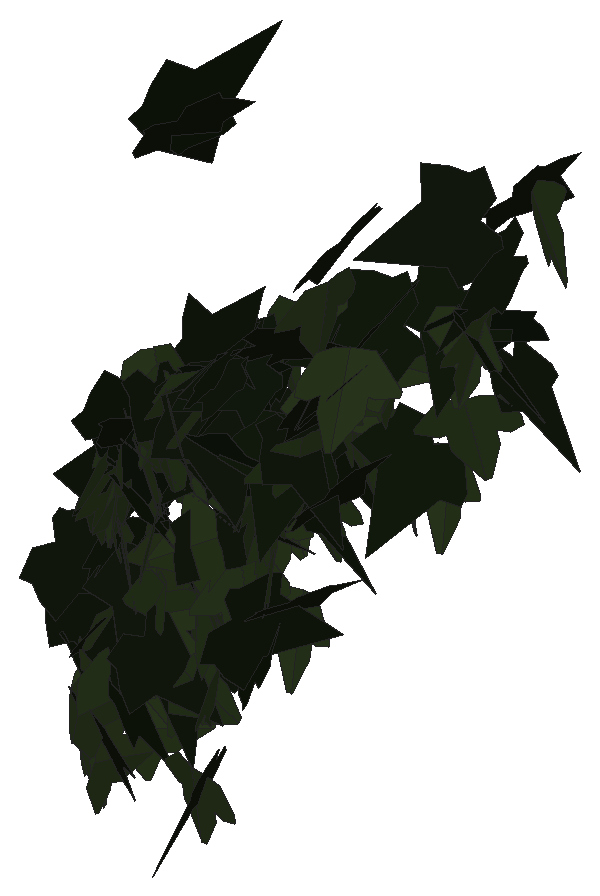
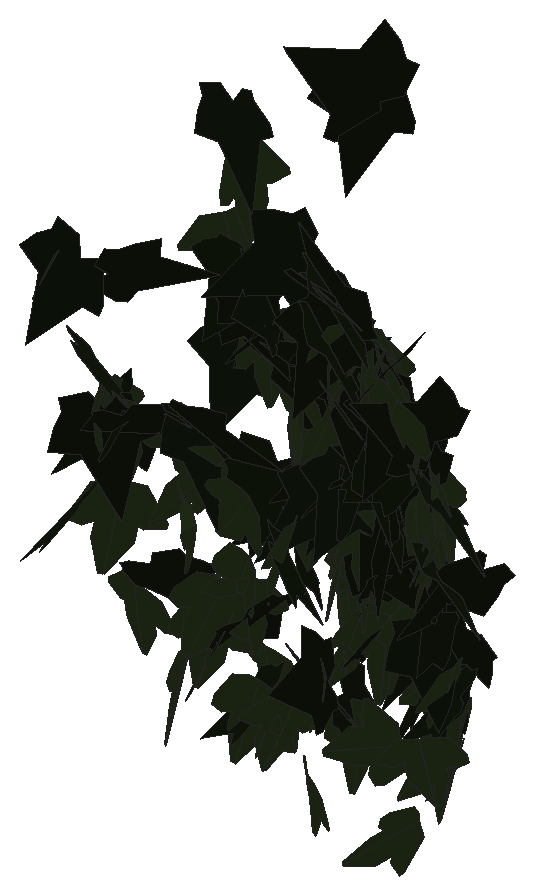
# SketchUp Ruby script. Lengths in inches.
U = 1.inch
M = Sketchup.active_model
def pt(a) = Geom::Point3d.new(a.map { |v| v * U })
def face(e, loops, mat)
  f = e.add_face(loops[0].map { |a| pt(a) })
  loops[1..].each { |l| e.add_face(l.map { |a| pt(a) }).erase! }
  f.material = f.back_material = mat if mat
  f
end
# faces: each face lists its corners as indices into pts; further lists are holes
def faces(e, pts, list, mat = nil) = list.each { |f| face(e, (f[0].is_a?(Array) ? f : [f]).map { |l| l.map { |i| pts[i] } }, mat) }
# xy, xz, yz: faces in a plane at the given z, y or x. An outline is a flat list of corners, or four numbers for a rectangle; further outlines are holes
def ring(l) = l.size == 4 ? [[l[0], l[1]], [l[2], l[1]], [l[2], l[3]], [l[0], l[3]]] : l.each_slice(2).to_a
def flat(e, list, mat, &to3) = list.each { |f| face(e, (f[0].is_a?(Array) ? f : [f]).map { |l| ring(l).map { |u, v| to3.(u, v) } }, mat) }
def xy(e, z, list, mat = nil) = flat(e, list, mat) { |x, y| [x, y, z] }
def xz(e, y, list, mat = nil) = flat(e, list, mat) { |x, z| [x, y, z] }
def yz(e, x, list, mat = nil) = flat(e, list, mat) { |y, z| [x, y, z] }
def lines(e, pts, list) = list.each { |a, b| e.add_line(pt(pts[a]), pt(pts[b])) }
# prism: a flat outline (further loops are holes) pulled along v
def prism(e, loops, v, mat = nil)
  f = face(e, loops, mat); d = Geom::Vector3d.new(v.map { |x| x * U })
  f.pushpull(f.normal.samedirection?(d) ? d.length : -d.length)
end
def box(e, o, s, mat = nil) = prism(e, [[o, [o[0] + s[0], o[1], o[2]], [o[0] + s[0], o[1] + s[1], o[2]], [o[0], o[1] + s[1], o[2]]]], [0, 0, s[2]], mat)
def at(x, y, z, deg = 0) = Geom::Transformation.translation(pt([x, y, z])) * Geom::Transformation.rotation(ORIGIN, Z_AXIS, deg.degrees)
def axes(o, x, y, z) = Geom::Transformation.new([*x, 0, *y, 0, *z, 0, *pt(o).to_a, 1])
def part(name) = M.definitions.add(name)
# library, detail: a bought-in or finely detailed component or shape, given as its bounding box
def library(name, o, s) = part(name).tap { |d| box(d.entities, o, s) }
def detail(e, o, s) = box(e.add_group.entities, o, s)
def put(e, d, t, mat = nil) = e.add_instance(d, t).tap { |i| i.material = mat if mat }
def group(e, t, mat = nil) = e.add_group.tap { |g| g.transformation = t; g.material = mat if mat }.entities
root = M.entities
M.materials.add("efeu1").color = [18, 25, 13]
M.materials.add("efeu2").color = [43, 57, 29]
c1 = part("ivyleaf_10")
p = [[0,0.5,-0.03],[-0.0625,2.02,-0.43],[-0.19,2.01,-0.46],[-0.54,1.05,-0.29],[-0.52,0.625,-0.18],[-0.83,0.76,-0.28],
  [-1.16,0.64,-0.33],[-1.15,0.33,-0.24],[-0.77,-0.39,0.02],[-0.3,-0.51,0.16],[0.04,-0.48,0.23],[-0.02,2.01,-0.4375],
  [-0.06,2.01,-0.43],[0.04,-0.49,0.23],[0.67,-0.49,0.14],[1.38,0.36,-0.2],[1.375,0.51,-0.24],[0.81,0.65,-0.19],
  [0.62,0.59,-0.15],[0.6,1.09,-0.28],[0.5,1.23,-0.31]]
faces(c1.entities,p,[[0,1,2,3,4,5,6,7,8,9,10],[11,12,0,13,14,15,16,17,18,19,20]],"efeu2")
c2 = part("ivyleaf_9")
p = [[1.54,2.16,1.25],[1.36,2.04,1.19],[-0.21,0.99,0.68],[-0.71,1.11,0.82],[-0.85,0.86,0.67],[-0.8,0.17,0.21],
  [-0.9,-0.01,0.1],[-0.67,-0.16,-0.02],[-0.08,-0.08,-0.05],[-0.03,-0.6,-0.4],[0.65,-0.88,-0.66],[0.83,-0.6,-0.49],
  [1.29,-0.42,-0.43],[1.8125,-0.07,-0.26],[1.21,0.44,0.15]]
faces(c2.entities,p,[[0,1,2,3,4,5,6,7,8,9,10,11,12,13,14]],"efeu1")
put(root,c1,axes([559.02,133.74,220.0625],[-0.14078,-0.88216,-0.06887],[0.00264,0.06931,-0.89328],[0.88484,-0.14056,-0.00829]))
put(root,c2,axes([556.01,133.8125,216.23],[-0.26742,-0.68197,-0.50877],[0.17433,0.47808,-0.73246],[0.83279,-0.31907,-0.01004]))
put(root,c1,axes([555.16,133.6,216.0625],[-0.46039,0.75729,-0.00295],[-0.00102,-0.00407,-0.88625],[-0.7573,-0.46038,0.00299]))
put(root,c2,axes([554.58,133.77,216.25],[0.44166,-0.72964,-0.25832],[-0.05083,0.26943,-0.84793],[0.77235,0.43497,0.09191]))
put(root,c2,axes([553.01,133.48,207.98],[0.77653,-0.04593,-0.47015],[-0.46839,0.04255,-0.77778],[0.06131,0.90677,0.01268]))
put(root,c2,axes([556.24,133.74,215.02],[0.44606,-0.24546,0.70342],[0.69118,-0.16966,-0.4975],[0.27807,0.81547,0.10823]))
put(root,c2,axes([556.68,133.75,217.57],[-0.7001,0.49631,0.19101],[-0.23436,-0.00448,-0.84735],[-0.47737,-0.72567,0.13587]))
put(root,c2,axes([555.56,133.26,223.17],[0.31745,0.86349,0.0264],[0.0086,0.02496,-0.92],[-0.86385,0.31757,0.00054]))
put(root,c1,axes([555.84,133.78,213.01],[-0.41657,0.26358,0.71128],[-0.7577,-0.18299,-0.37595],[0.03589,-0.80372,0.31886]))
put(root,c1,axes([554.58,133.89,216],[0.68612,-0.55,-0.06522],[-0.05978,0.02969,-0.87924],[0.55061,0.68858,-0.01419]))
put(root,c2,axes([554.49,133.53,210.3],[0.30628,-0.50665,-0.6268],[-0.10287,0.64048,-0.56797],[0.79937,0.27654,0.16706]))
put(root,c1,axes([559.5,133.85,218.39],[0.57533,0.6599,-0.15884],[-0.14364,-0.08513,-0.87397],[-0.66337,0.59075,0.05149]))
put(root,c2,axes([557.15,134,217.61],[-0.83228,0.17303,0.21694],[-0.22414,-0.01484,-0.84808],[-0.16359,-0.85996,0.05829]))
put(root,c1,axes([554.92,133.88,216.13],[0.05452,-0.88445,-0.07136],[-0.01495,0.07057,-0.88607],[0.8872,0.05554,-0.01054]))
put(root,c1,axes([554.7,133.78,215.36],[-0.86039,0.19813,-0.04154],[0.02888,-0.0594,-0.88141],[-0.20037,-0.85934,0.05135]))
put(root,c2,axes([556.59,133.5,217.71],[-0.36519,0.75552,0.27273],[-0.19522,0.20713,-0.83519],[-0.77916,-0.40601,0.08143]))
put(root,c1,axes([555.77,134.02,215.96],[0.01771,-0.87373,0.07357],[0.04283,-0.07263,-0.87294],[0.87578,0.02123,0.04121]))
put(root,c1,axes([553.21,133.18,208.43],[-0.01588,-0.12607,-0.94432],[0.22937,0.91617,-0.12617],[0.92468,-0.22942,0.01508]))
put(root,c1,axes([558.2,133.92,215.96],[-0.29422,-0.83577,-0.04837],[0.01575,0.04574,-0.88605],[0.83702,-0.29465,-0.00033]))
put(root,c2,axes([557.0625,133.25,211.8],[0.18463,0.11111,-0.87116],[-0.14229,0.88223,0.08236],[0.86662,0.12118,0.19912]))
put(root,c2,axes([555.51,134.36,207.25],[-0.4534,0.18215,-0.71547],[0.52437,-0.5116,-0.46255],[-0.51972,-0.67509,0.15749]))
put(root,c2,axes([557.71,134.3,215.82],[-0.62927,-0.54802,-0.2724],[0.25922,0.11524,-0.83067],[0.55437,-0.67594,0.07922]))
put(root,c1,axes([553.04,134.125,213.8],[0.68555,-0.47728,0.27133],[0.27945,-0.07027,-0.82967],[0.47257,0.73393,0.09701]))
put(root,c2,axes([555.85,133.92,217.11],[-0.40881,0.31836,0.72354],[0.52322,-0.50162,0.51634],[0.59255,0.66258,0.04325]))
put(root,c2,axes([555.36,133.4,223.03],[0.04974,-0.1674,1.02834],[0.84248,0.61216,0.0589],[-0.61297,0.82778,0.16439]))
put(root,c2,axes([559.49,133.64,221.49],[-0.21307,0.87033,-0.00129],[-0.00352,-0.00219,-0.89602],[-0.87032,-0.21306,0.00394]))
put(root,c2,axes([558.02,134.09,216.23],[0.28564,-0.78976,-0.26353],[-0.01577,0.27343,-0.83651],[0.83242,0.27618,0.07458]))
put(root,c1,axes([554.2,134.08,213.01],[0.52099,-0.68456,-0.04577],[0.01079,0.06564,-0.85891],[0.686,0.51887,0.04827]))
put(root,c1,axes([557.15,134.125,212.92],[0.65814,-0.58268,0.02379],[0.08224,0.05722,-0.87361],[0.57733,0.65608,0.09733]))
put(root,c2,axes([553.68,134.08,213.27],[0.69129,-0.52178,0.14899],[0.1631,-0.03034,-0.86303],[0.51754,0.70652,0.07297]))
put(root,c1,axes([557.1,134.06,214.46],[0.791,-0.38237,0.07111],[0.17709,0.2106,-0.8374],[0.34627,0.76576,0.26581]))
put(root,c1,axes([555.58,134.01,216.61],[-0.62089,-0.58095,-0.19488],[0.17414,0.09871,-0.84907],[0.5875,-0.64322,0.04572]))
put(root,c1,axes([553.77,134.06,214.75],[-0.66137,0.53417,-0.20947],[0.16062,-0.1345,-0.85014],[-0.55083,-0.68059,0.00361]))
put(root,c2,axes([553.82,134.55,211.19],[-0.33057,-0.7898,-0.03349],[0.00699,0.03338,-0.85616],[0.79048,-0.33058,-0.00643]))
put(root,c1,axes([553.03,134.23,213.37],[0.10584,-0.86488,-0.05368],[0.00049,0.05414,-0.8713],[0.86654,0.1056,0.00705]))
put(root,c1,axes([552.74,134.24,213.6],[0.28483,-0.82276,-0.06216],[0.00374,0.06705,-0.8703],[0.82509,0.28372,0.02541]))
put(root,c1,axes([553.29,134.2,212.23],[-0.42915,0.70692,-0.22816],[0.09672,-0.20808,-0.82663],[-0.73651,-0.43924,0.02439]))
put(root,c1,axes([556.46,134.26,212.05],[-0.46345,-0.73351,-0.0827],[0.22842,-0.04965,-0.83966],[0.70193,-0.46815,0.21863]))
put(root,c1,axes([553.9375,134.27,211.125],[0.74229,-0.41948,-0.09639],[-0.07398,0.06497,-0.85238],[0.42401,0.74569,0.02003]))
put(root,c2,axes([554.34,134.52,209.54],[0.19775,-0.83605,0.00887],[0.0181,-0.00483,-0.85896],[0.8359,0.19789,0.0165]))
put(root,c2,axes([554.07,133.7,215.34],[0.54796,0.68663,0.03417],[0.006,0.03892,-0.87826],[-0.68746,0.54764,0.01957]))
put(root,c1,axes([555.82,134.11,209.73],[0.33239,-0.73908,-0.31298],[-0.0796,0.30673,-0.80886],[0.79866,0.33816,0.04964]))
put(root,c2,axes([551.95,134.36,210.28],[-0.21802,-0.23195,-0.79436],[0.73256,0.32799,-0.29684],[0.38491,-0.75562,0.115]))
put(root,c2,axes([553.3125,134.23,213.65],[0.38314,-0.14045,0.77192],[0.72584,-0.26273,-0.40807],[0.29791,0.82075,0.00147]))
put(root,c2,axes([551.9375,133.78,211.59],[0.27524,-0.21759,-0.79415],[-0.12243,0.81722,-0.26634],[0.81426,0.19642,0.2284]))
put(root,c2,axes([555.94,134.33,215.25],[-0.7695,0.40234,-0.05586],[0.05087,-0.02325,-0.86833],[-0.403,-0.77117,-0.00296]))
put(root,c2,axes([555.47,134.04,216.12],[0.51613,0.58276,-0.41597],[-0.28607,-0.30222,-0.77836],[-0.65635,0.58998,0.01215]))
put(root,c2,axes([557.34,133.73,218.27],[0.70153,0.27035,0.45747],[0.34897,0.33696,-0.73429],[-0.40072,0.76673,0.1614]))
put(root,c2,axes([556.37,134.04,216.84],[-0.45104,0.74102,0.15174],[-0.0897,0.12302,-0.8674],[-0.75106,-0.4597,0.01247]))
put(root,c2,axes([558.47,134.42,217.29],[-0.28592,0.66817,-0.49804],[0.20755,-0.45285,-0.72669],[-0.8071,-0.35315,-0.01044]))
put(root,c1,axes([554.21,134.05,210.53],[-0.24888,-0.22454,0.81622],[0.63832,0.50903,0.33467],[-0.55603,0.68486,0.01886]))
put(root,c2,axes([553.29,133.87,214.74],[-0.02517,-0.03366,0.87772],[0.74537,0.46373,0.03916],[-0.4647,0.74564,0.01527]))
put(root,c1,axes([552.13,134.35,207.68],[-0.16021,0.82154,-0.12098],[0.01395,-0.12053,-0.83696],[-0.83028,-0.16055,0.00928]))
put(root,c2,axes([558.07,133.82,212.36],[0.32931,0.80594,0.12343],[-0.18803,0.2046,-0.83427],[-0.79336,0.28605,0.24896]))
put(root,c1,axes([556.77,134.52,214.32],[0.27147,-0.82407,-0.00815],[-0.00469,0.00704,-0.86763],[0.82409,0.2715,-0.00226]))
put(root,c2,axes([555.46,134.41,213],[0.2239,-0.71473,-0.43281],[-0.11689,0.41688,-0.7489],[0.82735,0.25232,0.01132]))
put(root,c2,axes([554.68,134.0625,213.46],[-0.29931,0.79821,0.13763],[-0.02118,0.13896,-0.852],[-0.80971,-0.29869,-0.02859]))
put(root,c1,axes([553.19,134.49,213],[0.15148,-0.84444,-0.06332],[-0.00047,0.06424,-0.85785],[0.84681,0.15109,0.01085]))
put(root,c1,axes([555.24,134.39,210.74],[-0.75989,0.37137,0.1778],[-0.24515,-0.10825,-0.82167],[-0.3308,-0.77287,0.20052]))
put(root,c2,axes([553.68,134.33,214.125],[0.79096,-0.33008,0.15479],[0.19861,0.08003,-0.84421],[0.30573,0.80198,0.14795]))
put(root,c2,axes([558.99,133.86,215.16],[0.20768,0.79963,0.33369],[-0.0056,0.34437,-0.82175],[-0.86645,0.18944,0.08529]))
put(root,c2,axes([552.93,134.24,213.66],[-0.50617,0.64874,0.28351],[-0.21896,0.18798,-0.82107],[-0.67327,-0.54886,0.05388]))
put(root,c2,axes([553.04,134.37,212.12],[-0.58777,0.61618,0.06786],[-0.05826,0.03819,-0.85141],[-0.61716,-0.59044,0.01575]))
put(root,c2,axes([557.07,133.89,210.21],[0.05705,0.27212,0.82938],[-0.16237,0.81995,-0.25785],[-0.85764,-0.13714,0.10399]))
put(root,c2,axes([555.9,134.04,217.08],[0.59771,0.63776,-0.01348],[-0.00752,-0.01144,-0.87406],[-0.63785,0.59775,-0.00234]))
put(root,c1,axes([554.6,134.5,212.13],[-0.70784,-0.48872,-0.01651],[0.02346,-0.00492,-0.86],[0.48844,-0.70802,0.01737]))
put(root,c1,axes([555.1,134.42,206.79],[-0.82996,0.16103,0.1785],[-0.17366,0.04207,-0.8454],[-0.16624,-0.8479,-0.00804]))
put(root,c2,axes([554.43,134.64,211.96],[0.09059,0.26322,-0.81336],[-0.63022,-0.53209,-0.24239],[-0.57764,0.62181,0.1369]))
put(root,c1,axes([555.08,134.3125,209.23],[-0.03284,-0.68861,-0.52327],[0.33051,0.47391,-0.6444],[0.79923,-0.22428,0.24498]))
put(root,c2,axes([553.08,134.41,208.39],[0.6183,-0.36653,-0.46491],[-0.38197,0.26662,-0.71819],[0.45231,0.72619,0.02903]))
put(root,c1,axes([554.26,134.52,209.47],[-0.8362,0.14038,0.1333],[-0.13642,-0.00794,-0.84737],[-0.13735,-0.84672,0.03005]))
put(root,c2,axes([558.16,133.99,216.73],[0.16862,0.24229,0.83571],[0.03001,0.84913,-0.25223],[-0.86961,0.07629,0.15334]))
put(root,c1,axes([552.88,134.07,206.71],[0.02037,-0.34001,-0.84093],[0.1424,0.83191,-0.33291],[0.89582,-0.12451,0.07205]))
put(root,c1,axes([555.72,134.24,211.19],[-0.45036,0.52077,0.53425],[-0.33961,0.41255,-0.68842],[-0.6643,-0.56396,-0.01025]))
put(root,c1,axes([553.625,134.8125,215.81],[0.88482,-0.08092,0.52092],[0.52131,-0.01699,-0.88812],[0.07837,1.02663,0.02636]))
put(root,c1,axes([555.84,134.8125,214.23],[-0.16641,0.98973,0.28837],[0.00609,-0.29115,1.0028],[1.03087,0.16149,0.04063]))
put(root,c2,axes([558.92,133.98,217.38],[0.23107,0.68548,0.5111],[-0.01317,0.53222,-0.70785],[-0.85494,0.17707,0.14905]))
put(root,c1,axes([552.78,134.54,212.29],[-0.43124,0.74065,0.05517],[-0.01875,0.05292,-0.85699],[-0.74247,-0.43153,-0.0104]))
put(root,c2,axes([551.8,134.79,208.69],[0.62787,-0.56293,-0.03573],[0.02115,0.07691,-0.84025],[0.56367,0.62416,0.07132]))
put(root,c2,axes([554.28,134.49,212.67],[0.45324,0.00637,-0.73237],[-0.73017,0.0711,-0.45126],[0.05712,0.85833,0.04282]))
put(root,c1,axes([553.125,134.55,210.08],[-0.43663,-0.6273,-0.38671],[0.1966,0.33404,-0.76384],[0.71021,-0.47812,-0.0263]))
put(root,c1,axes([552.02,134.71,206.82],[-0.24368,0.81359,-0.01001],[-0.00411,-0.01168,-0.84927],[-0.81364,-0.24361,0.00729]))
put(root,c1,axes([552.17,134.7,209.02],[-0.13837,0.83743,0.04284],[0.00032,0.04347,-0.84875],[-0.83853,-0.13817,-0.0074]))
put(root,c2,axes([552.51,134.61,210.57],[0.87409,-0.12322,-0.31616],[-0.31112,0.05772,-0.88264],[0.13546,0.92772,0.01292]))
put(root,c2,axes([552.84,134.61,209.85],[-0.09249,0.83843,-0.1339],[0.00041,-0.13465,-0.8434],[-0.84906,-0.0914,0.01418]))
put(root,c2,axes([555.33,134.42,213.04],[0.18096,0.72038,0.44001],[0.03005,0.44422,-0.73964],[-0.84359,0.17036,0.06804]))
put(root,c2,axes([555.42,134.91,213.06],[0.83364,0.21997,0.0242],[-0.0401,0.24291,-0.82662],[-0.21763,0.79783,0.245]))
put(root,c1,axes([551.91,135.94,207.75],[0.71693,0.42634,-0.10284],[-0.08636,-0.05598,-0.83411],[-0.42998,0.7221,-0.00394]))
put(root,c1,axes([552.84,136.16,207.62],[0.24792,-0.07685,0.80375],[0.74045,0.3569,-0.19427],[-0.32196,0.76164,0.17213]))
put(root,c2,axes([554.87,136.3,208.81],[-0.22091,0.53378,0.63302],[-0.45607,0.46839,-0.55412],[-0.69111,-0.47972,0.16333]))
put(root,c1,axes([551.85,136.7,205.9375],[0.0446,-0.28403,-0.78881],[0.47017,0.66249,-0.21196],[0.69414,-0.43048,0.19426]))
put(root,c1,axes([555.39,137.36,209.65],[0.83616,-0.15349,0.13647],[0.13622,-0.01375,-0.85006],[0.15372,0.84711,0.01093]))
put(root,c2,axes([558.89,138.9,219.49],[-0.58058,-0.32676,0.61837],[-0.53259,-0.31434,-0.66615],[0.45332,-0.78781,0.00932]))
put(root,c2,axes([556.74,139.03,216.18],[-0.78343,-0.0887,0.43046],[-0.43152,-0.01164,-0.78777],[0.08337,-0.89383,-0.03246]))
put(root,c1,axes([552.53,139.17,210.89],[-0.34199,0.40064,-0.69592],[0.41565,-0.55886,-0.526],[-0.68706,-0.53752,0.02819]))
put(root,c2,axes([556.42,138.92,216.24],[-0.26905,0.8534,0.01063],[-0.00388,0.00993,-0.89481],[-0.85346,-0.26908,0.00072]))
put(root,c2,axes([553.46,139.5,214.2],[-0.66625,0.29278,-0.48853],[0.43792,-0.21737,-0.72749],[-0.36415,-0.79705,0.01895]))
put(root,c1,axes([558.42,139.67,216.42],[0.1561,-0.89623,0.09459],[0.00712,-0.09477,-0.90967],[0.90118,0.15599,-0.0092]))
put(root,c1,axes([554.43,139.71,215.14],[-0.68573,0.09576,-0.51688],[0.41894,-0.41361,-0.63243],[-0.31752,-0.75254,0.28182]))
put(root,c1,axes([558.05,139.55,216.3],[0.8791,-0.05705,0.01339],[0.02206,0.13566,-0.87026],[0.05429,0.86867,0.13679]))
put(root,c1,axes([553,139.79,210.13],[-0.03351,0.79231,-0.3833],[-0.02098,-0.38419,-0.79232],[-0.87991,-0.02102,0.03349]))
put(root,c2,axes([556.77,140.04,212.83],[-0.69283,-0.56153,-0.02279],[0.01047,0.02326,-0.89174],[0.5619,-0.69281,-0.01148]))
put(root,c1,axes([556,139.01,215.16],[0.06506,0.40628,0.79383],[0.05198,0.79286,-0.41004],[-0.89024,0.07599,0.03407]))
put(root,c2,axes([553.85,140.25,212.5],[-0.27505,-0.82833,0.16934],[-0.01758,-0.17243,-0.87202],[0.84528,-0.27313,0.03697]))
put(root,c1,axes([553.17,139.52,214.64],[-0.30034,0.79558,0.16934],[-0.06771,0.15543,-0.85035],[-0.81058,-0.30776,0.00829]))
put(root,c2,axes([558.15,139.67,216.38],[0.77119,-0.40597,-0.12666],[-0.0847,0.11041,-0.86961],[0.41675,0.77368,0.05764]))
put(root,c2,axes([557.52,140.2,216.65],[-0.51594,-0.673,-0.22751],[0.14519,0.17535,-0.84798],[0.69542,-0.53592,0.00825]))
put(root,c2,axes([558.82,140.16,217.99],[-0.80144,0.21462,-0.30086],[0.25263,-0.20621,-0.82008],[-0.26972,-0.83084,0.12582]))
put(root,c1,axes([554.31,139.86,213.49],[-0.74295,0.38886,-0.17377],[0.12486,-0.13518,-0.83637],[-0.4072,-0.75093,0.06058]))
put(root,c2,axes([552.24,139.24,210.93],[0.1541,0.23543,0.82329],[0.25502,0.78594,-0.27248],[-0.81744,0.28958,0.0702]))
put(root,c1,axes([554.17,140.02,213.02],[0.80402,0.37325,-0.09895],[-0.10705,-0.00414,-0.88548],[-0.371,0.81008,0.04107]))
put(root,c1,axes([557.94,139.92,214.15],[-0.71563,-0.52511,-0.14065],[0.12114,0.07263,-0.88753],[0.52996,-0.7257,0.01295]))
put(root,c1,axes([560,139.78,219.76],[-0.42996,0.80707,0.14351],[-0.04708,0.13748,-0.91417],[-0.81838,-0.43193,-0.02281]))
put(root,c2,axes([554.51,139.87,212.41],[0.59724,-0.43254,-0.50281],[-0.4041,0.29923,-0.73741],[0.52594,0.72109,0.00439]))
put(root,c1,axes([556,139.66,213.96],[0.34735,-0.27488,0.78256],[-0.56388,0.54392,0.44135],[-0.60827,-0.6612,0.03773]))
put(root,c1,axes([551.75,140.35,208.8],[0.63694,-0.44961,0.31681],[0.30207,-0.11914,-0.77639],[0.45964,0.70134,0.07122]))
put(root,c2,axes([553.42,140.18,210.47],[0.61258,-0.58574,0.00179],[0.06728,0.06779,-0.84215],[0.58187,0.60882,0.09549]))
put(root,c2,axes([558.26,140.03,216.43],[0.27041,0.71689,-0.42514],[-0.29609,-0.33517,-0.75352],[-0.77911,0.37619,0.13881]))
put(root,c2,axes([559.4,139.63,219.96],[0.28482,0.7494,0.3799],[0.13471,0.35522,-0.8017],[-0.82933,0.31506,0.00025]))
put(root,c1,axes([554.88,140.2,212.15],[-0.84453,-0.1361,-0.05055],[0.0472,0.02474,-0.85526],[0.13729,-0.84568,-0.01689]))
put(root,c1,axes([552.57,140.14,210.48],[0.33319,0.76213,0.286],[0.10688,0.2654,-0.83175],[-0.80698,0.34983,0.00792]))
put(root,c1,axes([556.8,140.52,212.19],[0.86226,-0.13101,0.18554],[0.18388,-0.0249,-0.87215],[0.13332,0.88164,0.00294]))
put(root,c1,axes([554.69,140.31,212.84],[-0.81428,-0.09115,-0.26165],[0.2582,0.04501,-0.81922],[0.10051,-0.8541,-0.01525]))
put(root,c1,axes([553.58,140.34,210.54],[-0.84351,0.0756,-0.06583],[0.06516,-0.01043,-0.84688],[-0.07618,-0.84601,0.00456]))
put(root,c2,axes([557.91,141.5,214.65],[0.5286,-0.70482,-0.18242],[-0.01867,0.21223,-0.87411],[0.72781,0.51735,0.11006]))
put(root,c1,axes([554.81,141.53,211.1875],[-0.55343,0.68034,0.10155],[-0.09,0.0576,-0.87638],[-0.68197,-0.55972,0.03325]))
